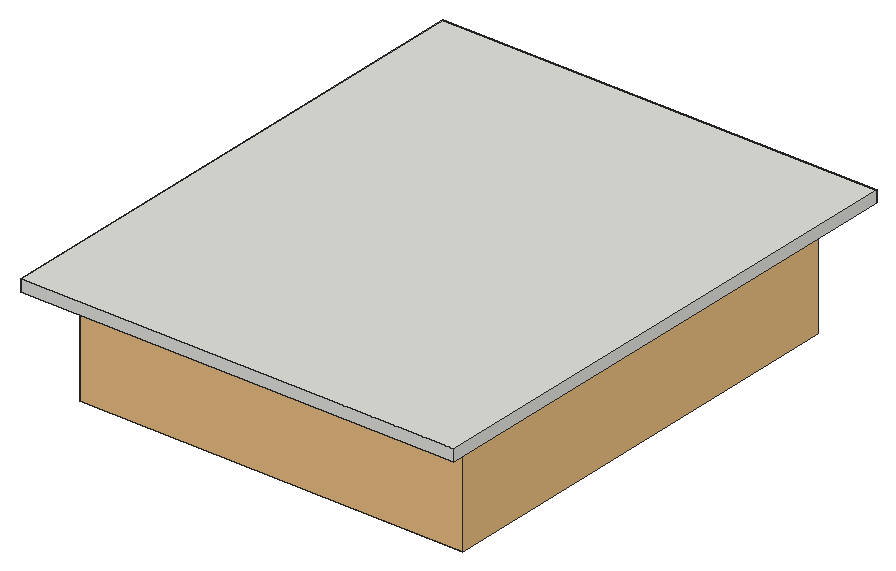
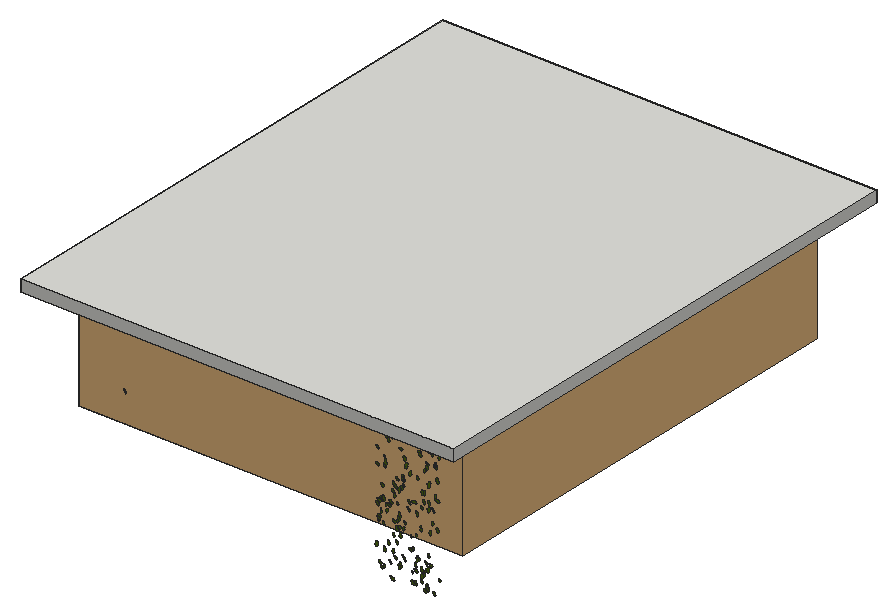
# SketchUp Ruby script. Lengths in inches.
U = 1.inch
M = Sketchup.active_model
def pt(a) = Geom::Point3d.new(a.map { |v| v * U })
def face(e, loops, mat)
  f = e.add_face(loops[0].map { |a| pt(a) })
  loops[1..].each { |l| e.add_face(l.map { |a| pt(a) }).erase! }
  f.material = f.back_material = mat if mat
  f
end
# faces: each face lists its corners as indices into pts; further lists are holes
def faces(e, pts, list, mat = nil) = list.each { |f| face(e, (f[0].is_a?(Array) ? f : [f]).map { |l| l.map { |i| pts[i] } }, mat) }
# xy, xz, yz: faces in a plane at the given z, y or x. An outline is a flat list of corners, or four numbers for a rectangle; further outlines are holes
def ring(l) = l.size == 4 ? [[l[0], l[1]], [l[2], l[1]], [l[2], l[3]], [l[0], l[3]]] : l.each_slice(2).to_a
def flat(e, list, mat, &to3) = list.each { |f| face(e, (f[0].is_a?(Array) ? f : [f]).map { |l| ring(l).map { |u, v| to3.(u, v) } }, mat) }
def xy(e, z, list, mat = nil) = flat(e, list, mat) { |x, y| [x, y, z] }
def xz(e, y, list, mat = nil) = flat(e, list, mat) { |x, z| [x, y, z] }
def yz(e, x, list, mat = nil) = flat(e, list, mat) { |y, z| [x, y, z] }
def lines(e, pts, list) = list.each { |a, b| e.add_line(pt(pts[a]), pt(pts[b])) }
# prism: a flat outline (further loops are holes) pulled along v
def prism(e, loops, v, mat = nil)
  f = face(e, loops, mat); d = Geom::Vector3d.new(v.map { |x| x * U })
  f.pushpull(f.normal.samedirection?(d) ? d.length : -d.length)
end
def box(e, o, s, mat = nil) = prism(e, [[o, [o[0] + s[0], o[1], o[2]], [o[0] + s[0], o[1] + s[1], o[2]], [o[0], o[1] + s[1], o[2]]]], [0, 0, s[2]], mat)
def at(x, y, z, deg = 0) = Geom::Transformation.translation(pt([x, y, z])) * Geom::Transformation.rotation(ORIGIN, Z_AXIS, deg.degrees)
def axes(o, x, y, z) = Geom::Transformation.new([*x, 0, *y, 0, *z, 0, *pt(o).to_a, 1])
def part(name) = M.definitions.add(name)
# library, detail: a bought-in or finely detailed component or shape, given as its bounding box
def library(name, o, s) = part(name).tap { |d| box(d.entities, o, s) }
def detail(e, o, s) = box(e.add_group.entities, o, s)
def put(e, d, t, mat = nil) = e.add_instance(d, t).tap { |i| i.material = mat if mat }
def group(e, t, mat = nil) = e.add_group.tap { |g| g.transformation = t; g.material = mat if mat }.entities
root = M.entities
M.materials.add("[Vegetation Blur 03]").color = [83, 114, 18]
c1 = library("Component\#7",[0,0,0],[4,4,1.1875])
c2 = library("Group\#117",[-5.38,-4.54,-0.11],[130.87,151.28,44.65])
c3 = library("Group\#45",[0,0,0],[130,167,2])
c4 = part("ivy")
xy(c4.entities,0,[[0.782,0,0.786,0,0.787,0.005,0.789,0.009,0.821,0.072,0.875,0.147,1.001,0.272,1.073,0.331,1.137,0.363,1.178,0.379,1.223,0.384,1.272,0.383,1.311,0.374,1.36,0.355,1.399,0.334,1.491,0.285,1.541,0.244,1.583,0.199,1.617,0.15,1.64,0.128,1.662,0.115,1.717,0.105,1.745,0.093,1.784,0.054,1.819,0.057,1.854,0.064,1.882,0.075,1.896,0.074,1.91,0.071,1.937,0.063,1.964,0.053,1.99,0.038,2.016,0.015,2.034,0.002,2.04,0,2.038,0.003,2.036,0.007,2.033,0.038,2.036,0.068,2.045,0.1,2.055,0.116,2.064,0.123,2.077,0.129,2.088,0.129,2.106,0.132,2.118,0.13,2.179,0.132,2.207,0.133,2.225,0.133,2.242,0.138,2.22,0.162,2.207,0.186,2.206,0.213,2.212,0.236,2.228,0.262,2.247,0.274,2.298,0.283,2.355,0.294,2.37,0.296,2.376,0.295,2.377,0.3,2.377,0.303,2.385,0.329,2.411,0.37,2.426,0.392,2.449,0.407,2.511,0.426,2.561,0.444,2.619,0.466,2.589,0.469,2.561,0.476,2.501,0.5,2.449,0.516,2.424,0.523,2.401,0.535,2.377,0.556,2.372,0.568,2.36,0.575,2.268,0.586,2.225,0.592,2.207,0.599,2.194,0.61,2.143,0.65,2.13,0.664,2.122,0.682,2.123,0.7,2.13,0.719,2.148,0.75,2.17,0.781,2.195,0.807,2.221,0.828,2.284,0.874,2.291,0.88,2.288,0.887,2.276,0.9,2.267,0.916,2.265,0.933,2.273,0.967,2.292,1.002,2.313,1.03,2.334,1.054,2.348,1.067,2.358,1.074,2.363,1.076,2.362,1.081,2.35,1.094,2.347,1.11,2.35,1.143,2.359,1.18,2.385,1.254,2.415,1.324,2.448,1.393,2.45,1.4,2.446,1.398,2.44,1.394,2.427,1.383,2.402,1.36,2.376,1.339,2.345,1.324,2.305,1.309,2.282,1.303,2.273,1.306,2.245,1.294,2.212,1.287,2.187,1.291,2.163,1.301,2.142,1.316,2.134,1.327,2.124,1.325,2.09,1.292,2.053,1.259,2.014,1.234,1.973,1.215,1.954,1.21,1.931,1.208,1.909,1.212,1.893,1.22,1.879,1.233,1.872,1.248,1.867,1.281,1.864,1.319,1.821,1.258,1.773,1.197,1.726,1.141,1.698,1.121,1.679,1.116,1.666,1.117,1.647,1.122,1.632,1.129,1.62,1.141,1.617,1.154,1.617,1.219,1.621,1.254,1.623,1.268,1.623,1.281,1.618,1.314,1.606,1.346,1.603,1.375,1.607,1.403,1.603,1.467,1.599,1.499,1.605,1.525,1.614,1.552,1.629,1.577,1.635,1.589,1.629,1.587,1.618,1.582,1.596,1.566,1.581,1.556,1.568,1.552,1.557,1.55,1.545,1.553,1.531,1.562,1.522,1.572,1.504,1.591,1.486,1.611,1.474,1.631,1.457,1.666,1.455,1.684,1.457,1.698,1.452,1.715,1.444,1.728,1.424,1.754,1.419,1.772,1.423,1.786,1.434,1.819,1.444,1.848,1.446,1.855,1.44,1.861,1.43,1.867,1.386,1.904,1.349,1.948,1.326,1.973,1.31,1.995,1.288,2.048,1.284,2.153,1.287,2.254,1.284,2.255,1.282,2.253,1.278,2.247,1.274,2.237,1.266,2.216,1.226,2.125,1.208,2.076,1.184,2.033,1.155,1.984,1.135,1.942,1.111,1.899,1.083,1.861,1.053,1.85,1.059,1.83,1.061,1.809,1.056,1.79,1.049,1.767,1.04,1.749,1.018,1.733,0.994,1.726,0.942,1.734,0.95,1.6875,0.944,1.645,0.932,1.608,0.911,1.585,0.881,1.58,0.854,1.582,0.828,1.588,0.785,1.618,0.773,1.625,0.775,1.614,0.779,1.598,0.796,1.502,0.818,1.402,0.861,1.283,0.882,1.224,0.894,1.174,0.892,1.148,0.886,1.123,0.881,1.107,0.872,1.099,0.849,1.094,0.818,1.092,0.789,1.098,0.762,1.107,0.753,1.113,0.721,1.139,0.698,1.163,0.678,1.194,0.665,1.224,0.628,1.28,0.612,1.312,0.606,1.327,0.606,1.314,0.599,1.282,0.594,1.267,0.581,1.256,0.544,1.245,0.512,1.244,0.473,1.249,0.444,1.256,0.382,1.288,0.339,1.306,0.324,1.316,0.317,1.324,0.309,1.326,0.27,1.314,0.227,1.313,0.185,1.3125,0.152,1.317,0.122,1.328,0.092,1.345,0.073,1.353,0.079,1.338,0.092,1.308,0.117,1.249,0.13,1.215,0.139,1.164,0.147,1.148,0.157,1.136,0.163,1.122,0.174,1.086,0.177,1.067,0.182,1.054,0.186,1.043,0.191,1.038,0.211,1.028,0.237,1.005,0.25,0.974,0.253,0.96,0.25,0.944,0.242,0.914,0.243,0.906,0.249,0.902,0.26,0.894,0.289,0.88,0.307,0.873,0.322,0.862,0.364,0.799,0.403,0.738,0.431,0.709,0.439,0.691,0.441,0.678,0.4375,0.66,0.428,0.645,0.394,0.623,0.303,0.594,0.255,0.581,0.214,0.577,0.179,0.573,0.173,0.568,0.175,0.561,0.167,0.55,0.141,0.523,0.113,0.503,0.077,0.49,0.045,0.486,0.026,0.485,0.019,0.486,0.011,0.483,0,0.471,0.014,0.467,0.044,0.455,0.058,0.447,0.07,0.438,0.097,0.411,0.125,0.394,0.158,0.377,0.174,0.366,0.182,0.359,0.185,0.361,0.242,0.331,0.253,0.316,0.258,0.303,0.262,0.283,0.274,0.278,0.308,0.274,0.341,0.252,0.366,0.226,0.366,0.222,0.37,0.22,0.38,0.221,0.395,0.221,0.425,0.216,0.45,0.207,0.465,0.192,0.473,0.178,0.484,0.15,0.489,0.116,0.483,0.089,0.468,0.058,0.45,0.035,0.435,0.018,0.429,0.011,0.434,0.012,0.438,0.014,0.469,0.019,0.542,0.016,0.581,0.015,0.612,0.027,0.68,0.055,0.696,0.057,0.712,0.052,0.73,0.045,0.741,0.036,0.766,0.014]])
box(root,[0,0,150],[148,180,4])
p = [[99.64,30.95,148],[99.56,30.9,148],[99,28.98,148],[99.04,28.9,148],[100.46,28.11,148],[100.56,28.125,148],
  [100.65,28.14,148],[100.74,28.16,148],[99.26,28.59,148],[99.33,28.52,148],[101.1,28.3,148],[101.18,28.35,148],
  [99.14,30.51,148],[99.09,30.4375,148],[99.26,30.66,148],[99.2,30.59,148],[99.8125,31.03,148],[99.72,30.99,148],
  [99.09,28.8125,148],[99.14,28.74,148],[99.2,28.66,148],[98.86,29.72,148],[98.85,29.625,148],[98.86,29.53,148],
  [99.4,28.46,148],[99.48,28.4,148],[98.93,30.09,148],[98.9,30,148],[100.08,28.14,148],[100.18,28.125,148],
  [98.87,29.81,148],[99.56,28.35,148],[99,30.27,148],[98.96,30.18,148],[99.48,30.85,148],[98.88,29.34,148],
  [98.9,29.25,148],[99.4,30.79,148],[99.33,30.73,148],[99.04,30.35,148],[99.64,28.3,148],[99.72,28.26,148],
  [98.87,29.44,148],[99.9,28.1875,148],[99.99,28.16,148],[99.8125,28.22,148],[100.37,28.11,148],[100.27,28.11,148],
  [100.84,28.1875,148],[100.93,28.22,148],[101.01,28.26,148],[98.93,29.16,148],[98.96,29.07,148],[98.88,29.91,148],
  [99.9,31.0625,148],[99.99,31.09,148],[101.88,29.53,148],[101.88,29.625,148],[101.65,28.8125,148],[101.69,28.9,148],
  [101.26,30.85,148],[101.18,30.9,148],[100.65,31.11,148],[100.56,31.125,148],[101.87,29.81,148],[101.85,29.91,148],
  [101.26,28.4,148],[101.33,28.46,148],[101.53,28.66,148],[101.59,28.74,148],[101.4,28.52,148],[101.88,29.72,148],
  [101.47,28.59,148],[101.83,30,148],[101.78,30.18,148],[101.74,30.27,148],[101.74,28.98,148],[101.65,30.4375,148],
  [101.59,30.51,148],[100.46,31.14,148],[100.37,31.14,148],[100.08,31.11,148],[100.18,31.125,148],[101.81,30.09,148],
  [101.78,29.07,148],[101.81,29.16,148],[101.83,29.25,148],[101.85,29.34,148],[101.69,30.35,148],[101.87,29.44,148],
  [100.27,31.14,148],[101.53,30.59,148],[101.47,30.66,148],[101.33,30.79,148],[100.84,31.0625,148],[100.74,31.09,148],
  [101.4,30.73,148],[101.1,30.95,148],[101.01,30.99,148],[100.93,31.03,148]]
lines(root,p,[[0,1],[2,3],[4,5],[5,6],[6,7],[8,9],[10,11],[12,13],[14,15],[16,17],[3,18],[19,20],
  [21,22],[22,23],[18,19],[24,25],[26,27],[28,29],[30,21],[25,31],[32,33],[1,34],[35,36],[33,26],
  [37,38],[15,12],[20,8],[39,32],[40,41],[23,42],[43,44],[44,28],[41,45],[46,4],[29,47],[7,48],
  [42,35],[17,0],[9,24],[31,40],[47,46],[34,37],[48,49],[49,50],[45,43],[50,10],[51,52],[27,53],
  [38,14],[13,39],[53,30],[36,51],[54,16],[52,2],[55,54],[56,57],[58,59],[60,61],[62,63],[64,65],
  [66,67],[68,69],[67,70],[57,71],[69,58],[72,68],[65,73],[74,75],[59,76],[77,78],[79,80],[81,55],
  [82,81],[83,74],[84,85],[86,87],[75,88],[85,86],[87,89],[80,90],[91,92],[88,77],[71,64],[70,72],
  [93,60],[78,91],[94,95],[96,93],[73,83],[95,62],[63,79],[76,84],[89,56],[97,98],[11,66],[99,94],
  [92,96],[90,82],[61,97],[98,99],[22,57]])
put(root,c1,at(46.02,27.48,147.8125))
put(root,c1,at(98.37,27.625,147.75))
put(root,c2,axes([13.29,19.86,112.72],[1,0,0],[0,1,0],[0,0,0.85]))
put(root,c3,at(9,9,148))
put(root,c1,at(45.79,110,147.6875))
put(root,c1,at(98.14,110.14,147.625))
put(root,c4,axes([12.45,173.2,127.39],[0.62306,-0.44776,0.08452],[0.0504,-0.33563,-0.52711],[-0.23565,-1.25564,0.11075]),"[Vegetation Blur 03]")
put(root,c4,axes([22.33,173.2,133.12],[0.43009,-0.41994,0.38446],[0.46829,-0.19735,-0.38284],[-0.21039,-1.29771,-0.06619]),"[Vegetation Blur 03]")
put(root,c4,axes([28.59,173.2,145],[0.61554,-0.40401,-0.01131],[-0.04771,-0.21545,-0.519],[-0.19095,-1.24853,0.09322]),"[Vegetation Blur 03]")
put(root,c4,axes([24.08,173.2,105.62],[0.09448,-0.24372,0.47773],[0.55916,-0.39227,-0.10514],[-0.20978,-1.15536,-0.06508]),"[Vegetation Blur 03]")
put(root,c4,axes([16.39,173.2,120.18],[0.48124,-0.36893,0.30519],[0.35516,-0.24188,-0.41903],[-0.21409,-1.23057,-0.00913]),"[Vegetation Blur 03]")
put(root,c4,axes([21.86,173.2,120.21],[0.50493,-0.24622,0.19162],[0.19585,-0.34808,-0.41408],[-0.17632,-1.09173,0.08881]),"[Vegetation Blur 03]")
put(root,c4,axes([27.23,173.2,107.01],[0.55698,-0.45746,-0.14027],[-0.2006,-0.09744,-0.48055],[-0.19678,-1.19551,0.09284]),"[Vegetation Blur 03]")
put(root,c4,axes([20.47,173.2,124.85],[0.61028,-0.27277,0.17175],[0.18054,-0.30337,-0.50308],[-0.17106,-1.2933,0.08178]),"[Vegetation Blur 03]")
put(root,c4,axes([30.97,173.2,117.76],[0.23423,-0.31556,0.37462],[0.44905,-0.24958,-0.22008],[-0.18046,-1.03065,-0.06141]),"[Vegetation Blur 03]")
put(root,c4,axes([23.9375,173.2,120.64],[0.40386,-0.35784,0.38449],[0.46593,-0.19708,-0.35483],[-0.18733,-1.26162,-0.05362]),"[Vegetation Blur 03]")
put(root,c4,axes([15.33,173.2,128.88],[0.58162,-0.37165,0.13863],[0.15197,-0.16988,-0.49633],[-0.1959,-1.23523,0.02655]),"[Vegetation Blur 03]")
put(root,c4,axes([22.72,173.2,133.63],[0.38011,-0.35457,0.334],[0.40396,-0.18413,-0.33696],[-0.18436,-1.13452,-0.04969]),"[Vegetation Blur 03]")
put(root,c4,axes([23.79,173.2,129.17],[0.29678,-0.27186,0.42657],[0.50911,-0.26247,-0.26224],[-0.17731,-1.20867,-0.039]),"[Vegetation Blur 03]")
put(root,c4,axes([31.75,173.2,140.81],[0.4979,-0.40473,-0.18477],[-0.2554,-0.09899,-0.42431],[-0.15719,-1.12116,0.10416]),"[Vegetation Blur 03]")
put(root,c4,axes([18.09,173.2,102.63],[0.29467,-0.10714,0.44848],[0.50944,-0.44068,-0.23951],[-0.21249,-1.20507,0.04772]),"[Vegetation Blur 03]")
put(root,c4,axes([13.66,173.2,134.14],[0.18149,-0.29755,0.51892],[0.63719,-0.20751,-0.16715],[-0.13848,-1.34475,-0.08903]),"[Vegetation Blur 03]")
put(root,c4,axes([23.22,173.2,106.5],[0.44878,-0.3413,0.36007],[0.4395,-0.14984,-0.38721],[-0.17027,-1.28634,-0.05043]),"[Vegetation Blur 03]")
put(root,c4,axes([16.04,173.2,131.1875],[0.25712,-0.18798,0.42224],[0.4923,-0.32764,-0.22263],[-0.18343,-1.14283,-0.00563]),"[Vegetation Blur 03]")
put(root,c4,axes([23.52,173.2,121.87],[0.47957,-0.26061,0.31785],[0.37221,-0.23733,-0.40467],[-0.1708,-1.24893,0.01057]),"[Vegetation Blur 03]")
put(root,c4,axes([28.98,173.2,125.38],[0.56286,-0.41503,0.17137],[0.21267,-0.05627,-0.48669],[-0.19885,-1.23496,-0.03542]),"[Vegetation Blur 03]")
put(root,c4,axes([10.12,173.2,144.42],[0.47356,-0.40672,0.26845],[0.33871,-0.06229,-0.41283],[-0.18036,-1.18486,-0.07045]),"[Vegetation Blur 03]")
put(root,c4,axes([30.84,173.2,118.9],[0.57824,-0.2854,0.09144],[0.09076,-0.20234,-0.48162],[-0.15346,-1.19504,0.05971]),"[Vegetation Blur 03]")
put(root,c4,axes([14.28,173.2,103.04],[0.3696,-0.27711,0.38105],[0.45779,-0.2062,-0.31935],[-0.16294,-1.2079,-0.0329]),"[Vegetation Blur 03]")
put(root,c4,axes([30.18,173.2,121.04],[0.31064,-0.27454,0.24989],[0.28954,-0.20759,-0.27561],[-0.1665,-0.87322,-0.01304]),"[Vegetation Blur 03]")
put(root,c4,axes([15.99,173.2,107.98],[0.55958,-0.3731,0.26041],[0.3198,-0.09162,-0.47837],[-0.18004,-1.32239,-0.04033]),"[Vegetation Blur 03]")
put(root,c4,axes([15.22,173.2,111.21],[0.5074,-0.4678,-0.2898],[-0.37384,0.02954,-0.44347],[-0.19497,-1.27408,0.09613]),"[Vegetation Blur 03]")
put(root,c4,axes([14.19,173.2,141.25],[0.5878,-0.24093,0.03931],[0.02588,-0.23212,-0.48155],[-0.12393,-1.19122,0.08588]),"[Vegetation Blur 03]")
put(root,c4,axes([28.25,173.2,136.22],[0.41734,-0.25524,0.42347],[0.50918,-0.21404,-0.35453],[-0.15923,-1.35344,-0.02379]),"[Vegetation Blur 03]")
put(root,c4,axes([31.02,173.2,122.98],[0.53293,-0.19106,0.2627],[0.2994,-0.28671,-0.43737],[-0.15029,-1.24869,0.06023]),"[Vegetation Blur 03]")
put(root,c4,axes([11.75,173.2,140.97],[0.11866,-0.26117,0.39663],[0.48542,-0.20436,-0.1179],[-0.12904,-1.00894,-0.07879]),"[Vegetation Blur 03]")
put(root,c4,axes([10.48,173.2,121.76],[0.52711,-0.21147,0.33505],[0.39283,-0.25745,-0.4372],[-0.15742,-1.35053,0.03088]),"[Vegetation Blur 03]")
put(root,c4,axes([27.42,173.2,124.24],[0.61381,-0.2023,0.00115],[-0.01893,-0.26118,-0.49641],[-0.09648,-1.23581,0.10472]),"[Vegetation Blur 03]")
put(root,c4,axes([17.64,173.2,123.84],[0.18528,-0.05644,0.53215],[0.61865,-0.42892,-0.15063],[-0.2078,-1.32731,0.02605]),"[Vegetation Blur 03]")
put(root,c4,axes([12.65,173.2,144.48],[0.53111,-0.22481,0.11811],[0.12292,-0.23121,-0.43739],[-0.1333,-1.10892,0.06725]),"[Vegetation Blur 03]")
put(root,c4,axes([31.51,173.2,110.26],[0.31828,-0.32105,0.3684],[0.45752,-0.11523,-0.27908],[-0.137,-1.13071,-0.07616]),"[Vegetation Blur 03]")
put(root,c4,axes([13.65,173.2,129.41],[0.62179,-0.3866,0.07255],[0.08725,-0.03824,-0.53009],[-0.18864,-1.29198,-0.00602]),"[Vegetation Blur 03]")
put(root,c4,axes([25.77,173.2,128.55],[0.51632,-0.17161,0.26126],[0.29868,-0.283,-0.42241],[-0.14219,-1.21766,0.06135]),"[Vegetation Blur 03]")
put(root,c4,axes([14.99,173.2,107.69],[0.16819,-0.22664,0.32974],[0.39401,-0.21788,-0.15742],[-0.14187,-0.87383,-0.04627]),"[Vegetation Blur 03]")
put(root,c4,axes([30.16,173.2,105.62],[0.59208,-0.24793,0.06374],[0.06017,-0.19072,-0.48897],[-0.13036,-1.21404,0.0638]),"[Vegetation Blur 03]")
put(root,c4,axes([17.23,173.2,111.18],[0.5531,-0.30937,0.07702],[0.082,-0.11827,-0.46698],[-0.15743,-1.14854,0.02734]),"[Vegetation Blur 03]")
put(root,c4,axes([22.82,173.2,132.16],[0.42016,-0.3703,-0.17602],[-0.23818,-0.04638,-0.36333],[-0.14889,-0.97076,0.0845]),"[Vegetation Blur 03]")
put(root,c4,axes([21.89,173.2,108.75],[0.26152,-0.04302,0.44662],[0.5117,-0.42542,-0.20602],[-0.19512,-1.17335,0.05832]),"[Vegetation Blur 03]")
put(root,c4,axes([17.57,173.2,110.93],[0.62192,-0.51222,0.08279],[0.13225,0.12501,-0.54004],[-0.23401,-1.29066,-0.08517]),"[Vegetation Blur 03]")
put(root,c4,axes([13.16,173.2,110.91],[0.58633,-0.27865,-0.1062],[-0.1477,-0.14213,-0.48453],[-0.11598,-1.22771,0.08019]),"[Vegetation Blur 03]")
put(root,c4,axes([10.79,173.2,131.28],[0.64635,-0.1795,-0.0483],[-0.07498,-0.25102,-0.52154],[-0.0741,-1.31182,0.10641]),"[Vegetation Blur 03]")
put(root,c4,axes([24.36,173.2,132.9],[0.46976,-0.15316,0.21327],[0.23871,-0.28032,-0.3819],[-0.12977,-1.07007,0.06952]),"[Vegetation Blur 03]")
put(root,c4,axes([15.3125,173.2,131.25],[0.21062,-0.15839,0.41958],[0.49728,-0.27124,-0.18238],[-0.15148,-1.11064,-0.0153]),"[Vegetation Blur 03]")
put(root,c4,axes([27.3,173.2,112.1],[0.40591,-0.18014,0.3374],[0.39655,-0.24525,-0.33836],[-0.14603,-1.16675,0.01903]),"[Vegetation Blur 03]")
put(root,c4,axes([19.64,173.2,113.2],[0.43914,-0.29657,0.03896],[0.03337,-0.10478,-0.37595],[-0.14811,-0.90294,0.03083]),"[Vegetation Blur 03]")
put(root,c4,axes([24.66,173.2,117.45],[0.34584,-0.27967,0.31588],[0.38688,-0.124,-0.2994],[-0.13639,-1.06088,-0.04828]),"[Vegetation Blur 03]")
put(root,c4,axes([28.54,173.2,110.03],[0.57796,-0.29472,0.19025],[0.2281,-0.10009,-0.48593],[-0.15109,-1.27852,-0.00582]),"[Vegetation Blur 03]")
put(root,c4,axes([11.8,173.2,131.73],[0.12614,-0.2409,0.28031],[0.3435,-0.16191,-0.12485],[-0.11696,-0.73532,-0.06434]),"[Vegetation Blur 03]")
put(root,c4,axes([21.49,173.2,137.39],[0.07798,-0.22712,0.49701],[0.61066,-0.17712,-0.07655],[-0.10063,-1.25091,-0.0794]),"[Vegetation Blur 03]")
put(root,c4,axes([27.42,173.2,143.55],[0.32606,-0.15993,0.37004],[0.43652,-0.25327,-0.27342],[-0.14515,-1.12098,0.00898]),"[Vegetation Blur 03]")
put(root,c4,axes([21.76,173.2,140.07],[0.58958,-0.29849,0.19052],[0.22934,-0.09222,-0.49546],[-0.15145,-1.30163,-0.00859]),"[Vegetation Blur 03]")
put(root,c4,axes([18.16,173.2,108.37],[0.33688,-0.08622,0.33874],[0.38873,-0.33347,-0.27086],[-0.15137,-1.04826,0.0583]),"[Vegetation Blur 03]")
put(root,c4,axes([26.33,173.2,125.15],[0.58365,-0.1286,0.23072],[0.26562,-0.28309,-0.47237],[-0.11521,-1.30414,0.07979]),"[Vegetation Blur 03]")
put(root,c4,axes([24.55,173.2,113.51],[0.49387,-0.24848,0.14861],[0.17062,-0.13992,-0.41447],[-0.13648,-1.07408,0.01961]),"[Vegetation Blur 03]")
put(root,c4,axes([31.73,173.2,135.75],[0.44457,-0.30415,-0.24459],[-0.31847,-0.07486,-0.37092],[-0.10118,-1.10076,0.09281]),"[Vegetation Blur 03]")
put(root,c4,axes([17.27,173.2,144.4],[0.54958,-0.28156,-0.28314],[-0.3622,-0.10008,-0.45262],[-0.08884,-1.33367,0.09374]),"[Vegetation Blur 03]")
put(root,c4,axes([25.05,173.2,108.68],[0.45593,-0.14871,0.15697],[0.17169,-0.25336,-0.36992],[-0.11285,-0.98625,0.07136]),"[Vegetation Blur 03]")
put(root,c4,axes([29.96,173.2,124.92],[0.52102,-0.20474,0.04178],[0.03433,-0.18504,-0.42777],[-0.1065,-1.06132,0.06652]),"[Vegetation Blur 03]")
put(root,c4,axes([16.13,173.2,104.6],[0.49081,-0.25055,0.00673],[-0.00728,-0.13032,-0.40947],[-0.12182,-1.0017,0.05159]),"[Vegetation Blur 03]")
put(root,c4,axes([10.69,173.2,136.7],[0.32628,-0.20206,0.40603],[0.49033,-0.18475,-0.27691],[-0.12932,-1.21026,-0.02552]),"[Vegetation Blur 03]")
put(root,c4,axes([14.06,173.2,112.98],[0.30081,-0.15518,0.1985],[0.21889,-0.23826,-0.25024],[-0.13012,-0.75955,0.03794]),"[Vegetation Blur 03]")
put(root,c4,axes([11.91,173.2,102.41],[0.52824,-0.2088,0.07813],[0.0803,-0.17577,-0.43551],[-0.11407,-1.09065,0.05523]),"[Vegetation Blur 03]")
put(root,c4,axes([23.2,173.2,115.6875],[0.38346,-0.30784,0.36497],[0.45646,-0.05536,-0.32679],[-0.11835,-1.21097,-0.07784]),"[Vegetation Blur 03]")
put(root,c4,axes([30.52,173.2,124.58],[0.64177,-0.16774,0.0763],[0.07979,-0.21804,-0.52237],[-0.09498,-1.31665,0.07678]),"[Vegetation Blur 03]")
put(root,c4,axes([20.375,173.2,113.54],[0.50163,-0.24569,-0.26541],[-0.34021,-0.12729,-0.40976],[-0.06534,-1.2236,0.09592]),"[Vegetation Blur 03]")
put(root,c4,axes([117.19,173.7,127.39],[0.62306,-0.44776,0.08452],[0.0504,-0.33563,-0.52711],[-0.23565,-1.25564,0.11075]),"[Vegetation Blur 03]")
put(root,c4,axes([10.32,173.2,107.27],[0.44114,-0.2833,-0.10477],[-0.14493,-0.08165,-0.37173],[-0.12012,-0.94191,0.06374]),"[Vegetation Blur 03]")
put(root,c4,axes([14.9,173.2,102.19],[0.53858,-0.252,0.05397],[0.05479,-0.1161,-0.44944],[-0.12794,-1.11057,0.03474]),"[Vegetation Blur 03]")
put(root,c4,axes([24.8125,173.2,125.92],[0.4464,-0.35085,-0.18371],[-0.23796,-0.0009,-0.38487],[-0.15203,-1.02878,0.06299]),"[Vegetation Blur 03]")
put(root,c4,axes([19.18,173.2,112.97],[0.15407,-0.1087,0.33806],[0.39127,-0.27976,-0.13293],[-0.14585,-0.86534,0.00051]),"[Vegetation Blur 03]")
put(root,c4,axes([23.5,173.2,142.85],[0.51677,-0.16,-0.11108],[-0.14975,-0.2188,-0.41446],[-0.04632,-1.0777,0.10064]),"[Vegetation Blur 03]")
put(root,c4,axes([24.92,173.2,130.13],[0.31073,-0.06738,0.37222],[0.4328,-0.32267,-0.24985],[-0.14749,-1.08882,0.05101]),"[Vegetation Blur 03]")
put(root,c4,axes([15.56,173.2,107.26],[0.4884,-0.38994,-0.09349],[-0.11293,0.05241,-0.42733],[-0.19047,-1.03097,0.01363]),"[Vegetation Blur 03]")
put(root,c4,axes([19.17,173.2,128.56],[0.49181,-0.15671,-0.3315],[-0.41314,-0.21702,-0.39213],[0.00973,-1.29451,0.10587]),"[Vegetation Blur 03]")
put(root,c4,axes([16.17,173.2,127.01],[0.44605,-0.17185,0.11357],[0.12178,-0.19918,-0.36599],[-0.10728,-0.94065,0.05675]),"[Vegetation Blur 03]")
put(root,c4,axes([30.07,173.2,104.57],[0.42261,-0.28747,-0.1193],[-0.16204,-0.06467,-0.35783],[-0.12093,-0.91792,0.06257]),"[Vegetation Blur 03]")
put(root,c4,axes([13.75,173.2,126.62],[0.10022,-0.2222,0.4688],[0.57871,-0.13035,-0.09212],[-0.08191,-1.19279,-0.07727]),"[Vegetation Blur 03]")
put(root,c4,axes([18.02,173.2,117.9],[0.3651,-0.20886,0.13721],[0.15459,-0.14475,-0.30864],[-0.12111,-0.81437,0.01967]),"[Vegetation Blur 03]")
put(root,c4,axes([22.19,173.2,133.11],[0.28904,-0.06987,0.39444],[0.46239,-0.30604,-0.23421],[-0.14468,-1.11768,0.03947]),"[Vegetation Blur 03]")
put(root,c4,axes([25.91,173.2,102.21],[0.65317,-0.15035,0.08957],[0.09783,-0.2124,-0.5313],[-0.08838,-1.34629,0.07382]),"[Vegetation Blur 03]")
put(root,c4,axes([18.89,173.2,102.98],[0.51611,-0.14167,0.29822],[0.35265,-0.22138,-0.42305],[-0.1179,-1.28232,0.04009]),"[Vegetation Blur 03]")
put(root,c4,axes([13.24,173.2,119.81],[0.1731,-0.14266,0.38005],[0.45428,-0.21748,-0.15066],[-0.12362,-0.99891,-0.02148]),"[Vegetation Blur 03]")
put(root,c4,axes([28.95,173.2,104.52],[0.23742,-0.1267,0.33587],[0.39552,-0.23419,-0.20013],[-0.12927,-0.94922,0.00454]),"[Vegetation Blur 03]")
put(root,c4,axes([20.01,173.2,135.72],[0.30187,-0.29092,0.34167],[0.43037,-0.04293,-0.25902],[-0.10016,-1.06123,-0.08319]),"[Vegetation Blur 03]")
put(root,c4,axes([30.4,173.2,119.55],[0.46252,-0.08041,0.20679],[0.23593,-0.28736,-0.36906],[-0.10033,-1.0465,0.08545]),"[Vegetation Blur 03]")
put(root,c4,axes([17.5625,173.2,135.49],[0.34266,-0.16677,0.2483],[0.29126,-0.18349,-0.28712],[-0.11956,-0.92493,0.01219]),"[Vegetation Blur 03]")
put(root,c4,axes([28.84,173.2,135.36],[0.35292,-0.17211,0.08002],[0.07901,-0.17569,-0.29156],[-0.10181,-0.73298,0.0511]),"[Vegetation Blur 03]")
put(root,c4,axes([18.13,173.2,107.41],[0.56213,-0.17838,-0.00831],[-0.02255,-0.16495,-0.45927],[-0.08432,-1.14512,0.06745]),"[Vegetation Blur 03]")
put(root,c4,axes([13.71,173.2,112.9],[0.37075,-0.20222,0.27738],[0.33431,-0.13128,-0.31269],[-0.11578,-1.02663,-0.01465]),"[Vegetation Blur 03]")
put(root,c4,axes([19.77,173.2,116.86],[0.29156,-0.09126,0.22735],[0.25627,-0.25873,-0.23525],[-0.11785,-0.78843,0.05088]),"[Vegetation Blur 03]")
put(root,c4,axes([15.98,173.2,105.65],[0.28606,-0.20547,0.36321],[0.44363,-0.1257,-0.24391],[-0.10592,-1.08138,-0.04066]),"[Vegetation Blur 03]")
put(root,c4,axes([29.75,173.2,124.59],[0.31137,-0.19726,0.4006],[0.48849,-0.13513,-0.26337],[-0.10722,-1.1885,-0.03655]),"[Vegetation Blur 03]")
put(root,c4,axes([14.26,173.2,140.08],[0.56579,-0.26175,0.06944],[0.08066,-0.05979,-0.47321],[-0.13005,-1.17586,0.0086]),"[Vegetation Blur 03]")
put(root,c4,axes([25.62,173.2,130.95],[0.39018,-0.19806,0.28181],[0.33951,-0.13277,-0.32778],[-0.115,-1.06391,-0.01155]),"[Vegetation Blur 03]")
put(root,c4,axes([29.53,173.2,129.7],[0.59158,-0.31026,-0.0564],[-0.07139,-0.00087,-0.49803],[-0.1497,-1.22563,0.01463]),"[Vegetation Blur 03]")
put(root,c4,axes([13.95,173.2,102.4],[0.19741,-0.09695,0.50499],[0.60705,-0.24693,-0.16553],[-0.12869,-1.3135,-0.00615]),"[Vegetation Blur 03]")
put(root,c4,axes([12.46,173.2,123.2],[0.23432,-0.21265,0.28086],[0.3439,-0.11223,-0.20448],[-0.10411,-0.84934,-0.0433]),"[Vegetation Blur 03]")
put(root,c4,axes([25.36,173.2,119.98],[0.58607,-0.17658,0.01299],[0.00501,-0.15402,-0.47969],[-0.08713,-1.19658,0.05983]),"[Vegetation Blur 03]")
put(root,c4,axes([28.97,173.2,138.2],[0.24496,-0.07431,0.21292],[0.23492,-0.26987,-0.19483],[-0.11909,-0.6852,0.05364]),"[Vegetation Blur 03]")
put(root,c4,axes([24.52,173.2,119.75],[0.21308,-0.12887,0.25392],[0.29486,-0.2048,-0.18116],[-0.11737,-0.74847,0.00585]),"[Vegetation Blur 03]")
put(root,c4,axes([14.07,173.2,108.14],[0.09309,-0.2572,0.47512],[0.59358,-0.05541,-0.08218],[-0.0469,-1.21192,-0.09707]),"[Vegetation Blur 03]")
put(root,c4,axes([25.66,173.2,114.98],[0.16191,-0.03187,0.41572],[0.48687,-0.31523,-0.1301],[-0.15054,-1.05373,0.02635]),"[Vegetation Blur 03]")
put(root,c4,axes([22.89,173.2,130.96],[0.51145,-0.25079,0.06105],[0.06998,-0.0596,-0.42899],[-0.12471,-1.06199,0.00966]),"[Vegetation Blur 03]")
put(root,c4,axes([20.92,173.2,128.05],[0.48032,-0.40321,-0.3461],[-0.42858,0.11763,-0.41773],[-0.18586,-1.31325,0.06885]),"[Vegetation Blur 03]")
put(root,c4,axes([11.86,173.2,141.49],[0.45619,-0.27219,-0.21417],[-0.27378,-0.03129,-0.38217],[-0.10679,-1.08253,0.0649]),"[Vegetation Blur 03]")
put(root,c4,axes([19.4375,173.2,106.15],[0.27567,-0.18278,0.07916],[0.08,-0.13493,-0.23455],[-0.1044,-0.58604,0.02931]),"[Vegetation Blur 03]")
put(root,c4,axes([15.24,173.2,138.58],[0.31604,-0.28517,0.16056],[0.20748,-0.01555,-0.27638],[-0.12189,-0.7659,-0.05417]),"[Vegetation Blur 03]")
put(root,c4,axes([25.36,173.2,127.4375],[0.37901,-0.24998,0.16924],[0.20826,-0.05609,-0.32368],[-0.11995,-0.88726,-0.02722]),"[Vegetation Blur 03]")
put(root,c4,axes([26.3,173.2,144.75],[0.0835,-0.00667,0.46395],[0.54474,-0.33722,-0.06606],[-0.16259,-1.13325,0.01693]),"[Vegetation Blur 03]")
put(root,c4,axes([13.7,173.2,144.87],[0.27432,-0.11887,0.39101],[0.46845,-0.2067,-0.22879],[-0.11587,-1.1171,0.00072]),"[Vegetation Blur 03]")
put(root,c4,axes([23.67,173.2,118.82],[0.56324,-0.31646,-0.09717],[-0.11977,0.02711,-0.47626],[-0.15324,-1.18433,0.01506]),"[Vegetation Blur 03]")
put(root,c4,axes([28.17,173.2,121.57],[0.07402,-0.1812,0.31745],[0.39109,-0.12634,-0.07209],[-0.07805,-0.80492,-0.06015]),"[Vegetation Blur 03]")
put(root,c4,axes([22.4,173.2,118.17],[0.15681,-0.19135,0.27864],[0.34217,-0.11382,-0.14055],[-0.09017,-0.7647,-0.0488]),"[Vegetation Blur 03]")
put(root,c4,axes([25.76,173.2,109.8125],[0.12637,-0.06641,0.44261],[0.52763,-0.25805,-0.10643],[-0.12947,-1.11645,-0.00173]),"[Vegetation Blur 03]")
put(root,c4,axes([16.43,173.2,142.66],[0.3032,0.00804,0.42723],[0.50376,-0.343,-0.23711],[-0.14236,-1.19666,0.07083]),"[Vegetation Blur 03]")
put(root,c4,axes([22.62,173.2,109.79],[0.24227,-0.06001,0.24324],[0.27574,-0.26297,-0.19314],[-0.11679,-0.74533,0.04856]),"[Vegetation Blur 03]")
put(root,c4,axes([11.36,173.2,141.6],[0.40522,-0.15446,0.13943],[0.15914,-0.15283,-0.3347],[-0.09744,-0.89194,0.0332]),"[Vegetation Blur 03]")
put(root,c4,axes([29.1875,173.2,117.59],[0.33061,-0.13828,0.23143],[0.27228,-0.16795,-0.27487],[-0.10387,-0.88042,0.01609]),"[Vegetation Blur 03]")
put(root,c4,axes([28.44,173.2,123.51],[0.18332,-0.13201,0.23981],[0.28131,-0.17522,-0.15841],[-0.10639,-0.6908,-0.00565]),"[Vegetation Blur 03]")
